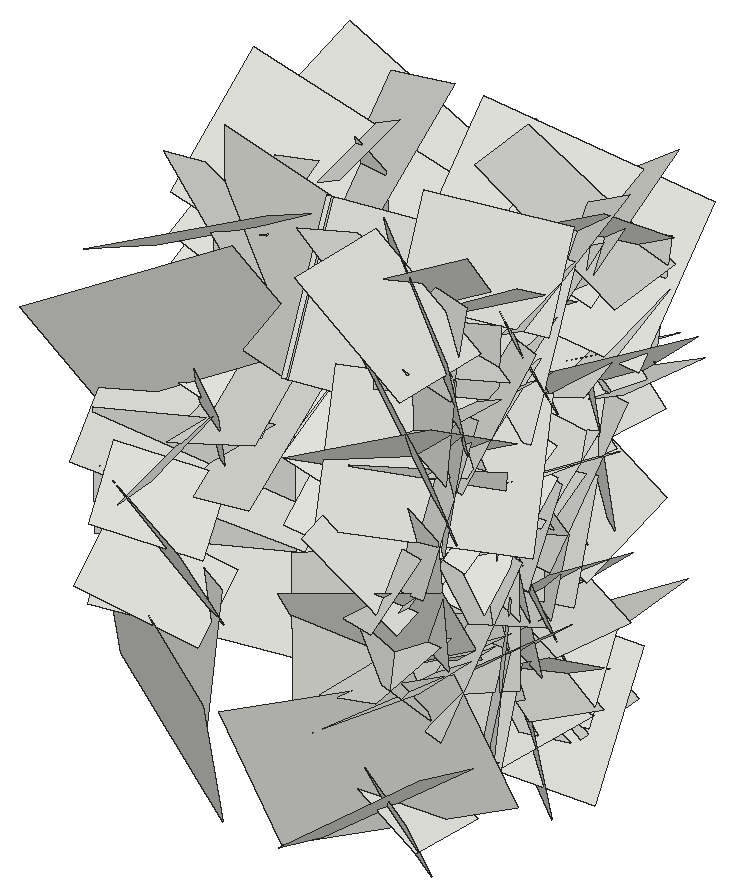
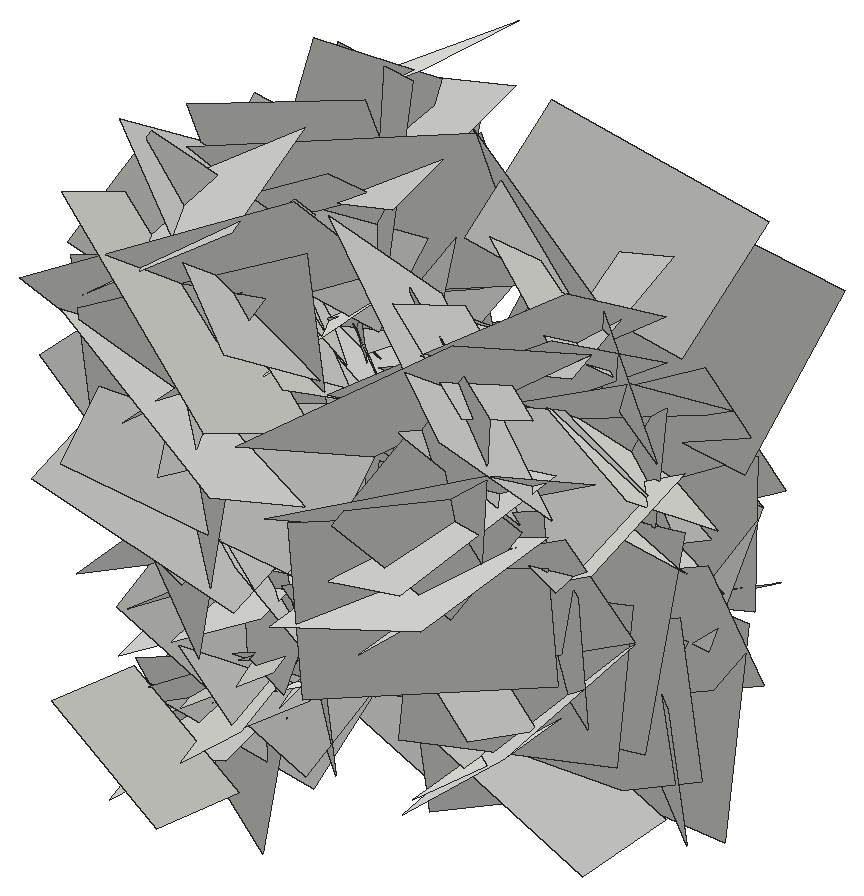
# SketchUp Ruby script. Lengths in inches.
U = 1.inch
M = Sketchup.active_model
def pt(a) = Geom::Point3d.new(a.map { |v| v * U })
def face(e, loops, mat)
  f = e.add_face(loops[0].map { |a| pt(a) })
  loops[1..].each { |l| e.add_face(l.map { |a| pt(a) }).erase! }
  f.material = f.back_material = mat if mat
  f
end
# faces: each face lists its corners as indices into pts; further lists are holes
def faces(e, pts, list, mat = nil) = list.each { |f| face(e, (f[0].is_a?(Array) ? f : [f]).map { |l| l.map { |i| pts[i] } }, mat) }
# xy, xz, yz: faces in a plane at the given z, y or x. An outline is a flat list of corners, or four numbers for a rectangle; further outlines are holes
def ring(l) = l.size == 4 ? [[l[0], l[1]], [l[2], l[1]], [l[2], l[3]], [l[0], l[3]]] : l.each_slice(2).to_a
def flat(e, list, mat, &to3) = list.each { |f| face(e, (f[0].is_a?(Array) ? f : [f]).map { |l| ring(l).map { |u, v| to3.(u, v) } }, mat) }
def xy(e, z, list, mat = nil) = flat(e, list, mat) { |x, y| [x, y, z] }
def xz(e, y, list, mat = nil) = flat(e, list, mat) { |x, z| [x, y, z] }
def yz(e, x, list, mat = nil) = flat(e, list, mat) { |y, z| [x, y, z] }
def lines(e, pts, list) = list.each { |a, b| e.add_line(pt(pts[a]), pt(pts[b])) }
# prism: a flat outline (further loops are holes) pulled along v
def prism(e, loops, v, mat = nil)
  f = face(e, loops, mat); d = Geom::Vector3d.new(v.map { |x| x * U })
  f.pushpull(f.normal.samedirection?(d) ? d.length : -d.length)
end
def box(e, o, s, mat = nil) = prism(e, [[o, [o[0] + s[0], o[1], o[2]], [o[0] + s[0], o[1] + s[1], o[2]], [o[0], o[1] + s[1], o[2]]]], [0, 0, s[2]], mat)
def at(x, y, z, deg = 0) = Geom::Transformation.translation(pt([x, y, z])) * Geom::Transformation.rotation(ORIGIN, Z_AXIS, deg.degrees)
def axes(o, x, y, z) = Geom::Transformation.new([*x, 0, *y, 0, *z, 0, *pt(o).to_a, 1])
def part(name) = M.definitions.add(name)
# library, detail: a bought-in or finely detailed component or shape, given as its bounding box
def library(name, o, s) = part(name).tap { |d| box(d.entities, o, s) }
def detail(e, o, s) = box(e.add_group.entities, o, s)
def put(e, d, t, mat = nil) = e.add_instance(d, t).tap { |i| i.material = mat if mat }
def group(e, t, mat = nil) = e.add_group.tap { |g| g.transformation = t; g.material = mat if mat }.entities
root = M.entities
c1 = part("Component\#6")
p = [[0.01,0,0],[0,3.24,4.54],[4.32,3.24,4.54],[4.33,0,0]]
faces(c1.entities,p,[[0,1,2,3]])
put(root,c1,axes([400.91,182.25,27.43],[-0.1955,0.46825,-1.21407],[0.10064,-1.21809,-0.48422],[1.37564,0.15566,-0.13711]))
put(root,c1,axes([414.68,182.25,27.43],[0.1955,0.46825,-1.21407],[-0.10064,-1.21809,-0.48422],[-1.37564,0.15566,-0.13711]))
put(root,c1,axes([414.68,183.5625,38.07],[-0.03427,-0.86867,-0.02883],[0.01016,-0.0292,0.8692],[-0.92124,0.03199,0.01066]))
put(root,c1,axes([404.88,183.51,30.36],[0.10644,-0.42009,-0.4575],[-0.01901,-0.46521,0.42323],[-0.65811,-0.0545,-0.08622]))
put(root,c1,axes([410.71,183.51,30.36],[-0.10644,-0.42009,-0.4575],[0.01901,-0.46521,0.42323],[0.65811,-0.0545,-0.08622]))
put(root,c1,axes([404.88,179.78,31.84],[0.01485,0.68647,0.23212],[0.1576,0.2245,-0.67291],[-0.75179,0.06062,-0.13648]))
put(root,c1,axes([410.71,179.78,31.84],[-0.01485,0.68647,0.23212],[-0.1576,0.2245,-0.67291],[0.75179,0.06062,-0.13648]))
put(root,c1,axes([400.91,181.64,30.57],[0.02444,0.48831,-0.77146],[0.19424,-0.75848,-0.47462],[0.9481,0.1428,0.11713]))
put(root,c1,axes([414.68,181.64,30.57],[-0.02444,0.48831,-0.77146],[-0.19424,-0.75848,-0.47462],[-0.9481,0.1428,0.11713]))
put(root,c1,axes([404.88,183.98,26.9],[0.15473,-0.64925,-0.29626],[-0.07231,-0.3137,0.65387],[-0.75301,-0.10329,-0.12366]))
put(root,c1,axes([410.71,183.98,26.9],[-0.15473,-0.64925,-0.29626],[0.07231,-0.3137,0.65387],[0.75301,-0.10329,-0.12366]))
put(root,c1,axes([410.71,181.88,29.24],[0.0732,0.47057,-0.46808],[-0.06498,-0.46407,-0.47558],[0.70054,-0.09222,0.00479]))
put(root,c1,axes([414.68,180.55,24.45],[-0.04702,0.95483,-0.28451],[0.08229,-0.28062,-0.95386],[-1.05288,-0.06457,-0.06184]))
put(root,c1,axes([410.71,182.11,23.57],[-0.01533,0.32032,-0.55846],[0.07998,-0.55391,-0.31966],[0.67773,0.07262,0.02509]))
put(root,c1,axes([400.91,182.41,31.86],[-0.21699,-0.67676,1.03332],[0.0082,1.04669,0.68705],[1.3093,-0.11872,0.16695]))
put(root,c1,axes([414.68,182.41,31.86],[0.21699,-0.67676,1.03332],[-0.0082,1.04669,0.68705],[-1.3093,-0.11872,0.16695]))
put(root,c1,axes([414.68,180.54,27.52],[-0.00647,0.86334,-0.00303],[0.00368,-0.003,-0.86336],[-0.91514,-0.00612,-0.00345]))
put(root,c1,axes([414.68,181.12,36.49],[0.0887,0.85058,-0.45713],[-0.14057,-0.44437,-0.85112],[-1.01388,0.13603,0.07801]))
put(root,c1,axes([410.71,184.65,28.76],[0.04824,-0.62434,-0.28052],[-0.09786,-0.28417,0.61748],[0.7189,0.00321,0.10288]))
put(root,c1,axes([414.68,185.4,30.76],[0.02152,-0.00963,-1.2106],[0.23963,-1.18945,0.01326],[-1.26071,-0.22625,-0.01814]))
put(root,c1,axes([410.71,181.75,22.9],[0.07496,0.59984,0.04506],[0.05269,0.03939,-0.60235],[0.63545,-0.07402,0.04463]))
put(root,c1,axes([400.91,185.55,26.35],[0.05433,-0.24183,-1.04679],[-0.06418,-1.04696,0.23891],[1.13701,-0.04754,0.0635]))
put(root,c1,axes([414.68,185.55,26.35],[-0.05433,-0.24183,-1.04679],[0.06418,-1.04696,0.23891],[-1.13701,-0.04754,0.0635]))
put(root,c1,axes([400.91,181.98,27.65],[0.03848,-0.07343,1.06513],[0.13392,1.05855,0.06867],[1.12376,-0.12364,-0.04466]))
put(root,c1,axes([414.68,181.98,27.65],[-0.03848,-0.07343,1.06513],[-0.13392,1.05855,0.06867],[-1.12376,-0.12364,-0.04466]))
put(root,c1,axes([410.71,184.92,37.05],[0.01613,-0.13323,-0.78421],[0.01491,-0.78419,0.1335],[0.84304,0.01642,0.01265]))
put(root,c1,axes([414.68,182.91,34.72],[0.14912,-0.41506,0.98502],[0.044,0.99488,0.41329],[-1.13217,-0.016,0.1458]))
put(root,c1,axes([410.71,184.84,39.1],[0.02023,-0.20369,-0.6632],[0.11732,-0.65406,0.20407],[0.72599,0.11137,-0.0145]))
put(root,c1,axes([410.71,182.78,23.92],[-0.06221,-0.24398,0.83625],[-0.07047,0.83695,0.23952],[0.92069,0.04758,0.07484]))
put(root,c1,axes([400.91,184.99,36.41],[0.13687,-0.99381,0.45239],[0.15227,0.46704,0.985],[1.14738,0.05657,-0.18469]))
put(root,c1,axes([414.68,184.99,36.41],[-0.13687,-0.99381,0.45239],[-0.15227,0.46704,0.985],[-1.14738,0.05657,-0.18469]))
put(root,c1,axes([414.68,184.8,33.37],[-0.19651,0.19461,-0.78555],[0.01158,-0.80522,-0.20206],[-0.85778,-0.05545,0.17724]))
put(root,c1,axes([414.68,187.08,35.11],[0.23629,-0.52338,-1.02054],[0.13084,-1.02265,0.55142],[-1.20867,-0.21302,-0.13982]))
put(root,c1,axes([410.71,183.74,37.84],[0.08456,-0.37494,0.46177],[-0.03825,0.46199,0.38136],[0.62935,0.07846,-0.03886]))
put(root,c1,axes([404.88,183.4375,30.23],[0.10865,-0.24445,0.66529],[-0.00738,0.67183,0.24793],[-0.75127,-0.04195,0.09378]))
put(root,c1,axes([410.71,183.4375,30.23],[-0.10865,-0.24445,0.66529],[0.00738,0.67183,0.24793],[0.75127,-0.04195,0.09378]))
put(root,c1,axes([400.91,180.73,30.67],[0.05707,0.69485,1.12415],[-0.04583,1.1254,-0.69356],[1.4001,0.00851,-0.06852]))
put(root,c1,axes([414.68,180.73,30.67],[-0.05707,0.69485,1.12415],[0.04583,1.1254,-0.69356],[-1.4001,0.00851,-0.06852]))
put(root,c1,axes([410.71,183.3,35.54],[0.06853,-0.0517,0.64839],[0.02911,0.65122,0.04919],[0.68886,-0.02238,-0.06659]))
put(root,c1,axes([410.71,186.27,36.66],[-0.23271,0.08267,-1.0169],[-0.17131,-1.02986,-0.04883],[1.06781,-0.14721,-0.22945]))
put(root,c1,axes([400.91,187.29,32.09],[-0.03087,-0.89426,-0.74249],[0.26998,-0.72958,0.86873],[1.20212,0.14089,-0.21417]))
put(root,c1,axes([414.68,187.29,32.09],[0.03087,-0.89426,-0.74249],[-0.26998,-0.72958,0.86873],[-1.20212,0.14089,-0.21417]))
put(root,c1,axes([400.91,187.26,33.24],[0.066,-0.95024,-0.64083],[0.19237,-0.6255,0.94515],[1.19957,0.15259,-0.11631]))
put(root,c1,axes([414.68,187.26,33.24],[-0.066,-0.95024,-0.64083],[-0.19237,-0.6255,0.94515],[-1.19957,0.15259,-0.11631]))
put(root,c1,axes([414.68,182.86,27.86],[-0.00866,0.87216,-0.09866],[-0.12421,-0.09886,-0.86427],[-0.92206,0.00513,0.11735]))
put(root,c1,axes([410.71,186.9,33.68],[-0.12726,-0.80704,-0.07778],[0.05104,-0.08559,0.81372],[0.85791,-0.11462,-0.05995]))
put(root,c1,axes([400.91,181.61,25.33],[-0.14764,0.72138,1.18272],[0.09804,1.19088,-0.71546],[1.46521,-0.007,0.16705]))
put(root,c1,axes([414.68,181.61,25.33],[0.14764,0.72138,1.18272],[-0.09804,1.19088,-0.71546],[-1.46521,-0.007,0.16705]))
put(root,c1,axes([414.68,186.8,27.07],[0.11611,-1.02809,0.5245],[0.14127,0.5346,1.02006],[-1.21522,-0.03608,0.16869]))
put(root,c1,axes([400.91,188.1875,39.24],[0.00053,-0.50504,-1.25708],[0.1621,-1.24903,0.50186],[1.42684,0.14209,-0.05655]))
put(root,c1,axes([414.68,188.1875,39.24],[-0.00053,-0.50504,-1.25708],[-0.1621,-1.24903,0.50186],[-1.42684,0.14209,-0.05655]))
put(root,c1,axes([400.91,182.88,33.98],[0.05541,0.90127,0.55592],[0.17138,0.54328,-0.89597],[1.1093,-0.12895,0.11065]))
put(root,c1,axes([414.68,182.88,33.98],[-0.05541,0.90127,0.55592],[-0.17138,0.54328,-0.89597],[-1.1093,-0.12895,0.11065]))
put(root,c1,axes([410.71,187.74,23.43],[-0.08523,-0.9506,0.05636],[-0.09187,0.06363,0.94959],[1.00521,-0.07479,0.09156]))
put(root,c1,axes([404.88,186.02,29.02],[0.12909,0.32312,-0.64935],[0.06195,-0.66067,-0.31779],[-0.76632,0.00102,-0.13508]))
put(root,c1,axes([410.71,186.02,29.02],[-0.12909,0.32312,-0.64935],[-0.06195,-0.66067,-0.31779],[0.76632,0.00102,-0.13508]))
put(root,c1,axes([414.68,182.62,33.52],[0.16113,0.63843,0.91206],[0.00988,0.91976,-0.64538],[-1.18006,0.09488,0.11913]))
put(root,c1,axes([410.71,187.61,26.86],[-0.07932,-0.16974,-0.83453],[-0.0041,-0.83766,0.17072],[0.9027,-0.01872,-0.07255]))
put(root,c1,axes([400.91,185.29,39.56],[0.11827,0.82487,-0.51088],[0.03346,-0.51706,-0.82795],[1.02793,-0.07808,0.08573]))
put(root,c1,axes([414.68,185.29,39.56],[-0.11827,0.82487,-0.51088],[-0.03346,-0.51706,-0.82795],[-1.02793,-0.07808,0.08573]))
put(root,c1,axes([410.71,188.3,31.13],[-0.1103,-0.11339,-0.88165],[-0.13763,-0.87621,0.12802],[0.93214,-0.14279,-0.08543]))
put(root,c1,axes([410.71,184.52,38.07],[-0.06477,0.36641,0.7198],[0.11209,0.71927,-0.35717],[0.84878,-0.06703,0.10209]))
put(root,c1,axes([414.68,184.16,23.6],[-0.00632,0.19994,1.20323],[0.15077,1.19515,-0.1979],[-1.28409,0.13934,-0.02916]))
put(root,c1,axes([400.91,184.16,23.6],[0.00632,0.19994,1.20323],[-0.15077,1.19515,-0.1979],[1.28409,0.13934,-0.02916]))
put(root,c1,axes([404.88,188.74,27.6],[0.13014,-0.45431,-0.37588],[0.00674,-0.3829,0.46487],[-0.62498,-0.09873,-0.07326]))
put(root,c1,axes([410.71,188.74,27.6],[-0.13014,-0.45431,-0.37588],[-0.00674,-0.3829,0.46487],[0.62498,-0.09873,-0.07326]))
put(root,c1,axes([410.71,188.62,32.29],[-0.0866,-0.74743,0.19758],[-0.06186,0.20408,0.74787],[0.81715,-0.06376,0.07755]))
put(root,c1,axes([404.88,185.35,37.93],[0.06077,0.5182,0.40006],[-0.00909,0.40215,-0.51968],[-0.69387,0.04012,0.04185]))
put(root,c1,axes([410.71,185.35,37.93],[-0.06077,0.5182,0.40006],[0.00909,0.40215,-0.51968],[0.69387,0.04012,0.04185]))
put(root,c1,axes([400.91,189.07,22.99],[0.09993,-0.91741,-0.05408],[0.10319,-0.04408,0.91762],[0.96866,0.09934,-0.09218]))
put(root,c1,axes([414.68,189.07,22.99],[-0.09993,-0.91741,-0.05408],[-0.10319,-0.04408,0.91762],[-0.96866,0.09934,-0.09218]))
put(root,c1,axes([400.91,186.51,25.44],[-0.00901,-0.3677,1.34811],[0.26845,1.32541,0.3631],[1.45667,-0.24653,-0.05858]))
put(root,c1,axes([414.68,186.51,25.44],[0.00901,-0.3677,1.34811],[-0.26845,1.32541,0.3631],[-1.45667,-0.24653,-0.05858]))
put(root,c1,axes([400.91,184.85,32.98],[-0.15473,1.07562,-0.16592],[0.16403,-0.14519,-1.07739],[1.14193,0.1666,0.13228]))
put(root,c1,axes([414.68,184.85,32.98],[0.15473,1.07562,-0.16592],[-0.16403,-0.14519,-1.07739],[-1.14193,0.1666,0.13228]))
put(root,c1,axes([400.91,189.26,31.29],[0.07003,-0.18149,-1.00879],[0.05402,-1.00905,0.18487],[1.08514,0.06195,0.0559]))
put(root,c1,axes([414.68,189.26,31.29],[-0.07003,-0.18149,-1.00879],[-0.05402,-1.00905,0.18487],[-1.08514,0.06195,0.0559]))
put(root,c1,axes([414.68,185.86,28.71],[0.06844,0.29244,0.76285],[-0.17475,0.75415,-0.27515],[-0.84819,-0.13178,0.11824]))
put(root,c1,axes([414.68,187.32,34.27],[-0.05201,-0.4187,0.7383],[0.02779,0.73844,0.42051],[-0.89926,0.04704,-0.0297]))
put(root,c1,axes([414.68,191.48,24.4],[0.24044,-0.84726,-0.84182],[0.11443,-0.83882,0.87332],[-1.26085,-0.2377,-0.08127]))
put(root,c1,axes([414.68,186.85,26],[-0.04759,0.74401,-0.43208],[-0.09551,-0.43435,-0.73856],[-0.90698,0.0067,0.10045]))
put(root,c1,axes([414.68,189.58,22.99],[0.08755,-0.94666,0.34405],[0.04779,0.34833,0.94763],[-1.06661,-0.0621,0.0707]))
put(root,c1,axes([414.68,186.99,20.26],[-0.04681,-0.17583,0.86867],[0.05724,0.86759,0.17835],[-0.93771,0.06173,-0.03248]))
put(root,c1,axes([400.91,190.19,31.82],[0.07854,-1.04848,0.11995],[-0.05802,0.11627,1.05008],[1.11713,0.07975,0.0461]))
put(root,c1,axes([414.68,190.19,31.82],[-0.07854,-1.04848,0.11995],[0.05802,0.11627,1.05008],[-1.11713,0.07975,0.0461]))
put(root,c1,axes([400.91,187.65,25.55],[0.14301,-0.32766,0.90945],[0.11586,0.91755,0.31436],[1.01811,-0.05839,-0.16352]))
put(root,c1,axes([414.68,187.65,25.55],[-0.14301,-0.32766,0.90945],[-0.11586,0.91755,0.31436],[-1.01811,-0.05839,-0.16352]))
put(root,c1,axes([400.91,186.92,28.87],[0.11772,1.08189,-0.3436],[-0.18933,-0.32428,-1.0788],[1.18826,-0.15885,-0.13785]))
put(root,c1,axes([414.68,186.92,28.87],[-0.11772,1.08189,-0.3436],[0.18933,-0.32428,-1.0788],[-1.18826,-0.15885,-0.13785]))
put(root,c1,axes([414.68,186.48,30.64],[-0.03295,0.70699,0.47041],[-0.18441,0.45544,-0.69599],[-0.88105,-0.12176,0.12808]))
put(root,c1,axes([400.91,185.59,36.56],[0.07365,1.00309,0.56692],[0.00038,0.56794,-1.00493],[1.22135,-0.06067,-0.03387]))
put(root,c1,axes([414.68,185.59,36.56],[-0.07365,1.00309,0.56692],[-0.00038,0.56794,-1.00493],[-1.22135,-0.06067,-0.03387]))
put(root,c1,axes([410.71,189.49,31],[-0.19159,0.03614,-0.77666],[0.1449,-0.78347,-0.06827],[0.81131,0.14846,-0.17121]))
put(root,c1,axes([414.68,189.24,21.76],[-0.15995,-0.688,0.38857],[0.02017,0.39231,0.70202],[-0.83731,0.14088,-0.05731]))
put(root,c1,axes([410.71,186.98,23.44],[-0.07046,0.41434,0.63319],[0.10971,0.63463,-0.40442],[0.79457,-0.05088,0.11199]))
put(root,c1,axes([414.68,190.89,25.45],[0.07637,-0.93381,0.1535],[-0.06656,0.14888,0.93522],[-1.00091,-0.08115,-0.05048]))
put(root,c1,axes([410.71,188.48,31.6],[0.00806,0.51701,-0.38199],[0.06142,-0.38101,-0.51453],[0.67861,0.02834,0.0511]))
put(root,c1,axes([400.91,185.63,37.94],[-0.10296,1.07287,0.66666],[-0.13207,0.65722,-1.07584],[1.33238,0.14805,-0.05512]))
put(root,c1,axes([414.68,185.63,37.94],[0.10296,1.07287,0.66666],[0.13207,0.65722,-1.07584],[-1.33238,0.14805,-0.05512]))
put(root,c1,axes([404.88,191.07,24.72],[0.08022,-0.60182,-0.03468],[0.03515,-0.03074,0.60586],[-0.63802,-0.07736,0.02902]))
put(root,c1,axes([410.71,191.07,24.72],[-0.08022,-0.60182,-0.03468],[-0.03515,-0.03074,0.60586],[0.63802,-0.07736,0.02902]))
put(root,c1,axes([414.68,187.18,35.87],[0.21905,1.32848,-0.23139],[0.18572,-0.25856,-1.32798],[-1.41727,0.17144,-0.20979]))
put(root,c1,axes([410.71,188.01,25.87],[-0.18323,0.88768,-0.1275],[-0.06793,-0.14175,-0.89995],[0.94816,0.16139,-0.08912]))
put(root,c1,axes([404.88,188.41,35.3125],[-0.03073,0.48255,0.4704],[0.10717,0.46862,-0.47449],[-0.70624,0.05011,-0.09248]))
put(root,c1,axes([410.71,188.41,35.3125],[0.03073,0.48255,0.4704],[-0.10717,0.46862,-0.47449],[0.70624,0.05011,-0.09248]))
put(root,c1,axes([400.91,186.91,28.91],[-0.08475,0.77289,1.06783],[0.0494,1.07079,-0.77154],[1.39641,0.00903,0.0921]))
put(root,c1,axes([414.68,186.91,28.91],[0.08475,0.77289,1.06783],[-0.0494,1.07079,-0.77154],[-1.39641,0.00903,0.0921]))
put(root,c1,axes([410.71,187.84,31.26],[0.01205,0.8882,0.30464],[-0.22592,0.29915,-0.86424],[0.96935,0.05868,-0.20521]))
put(root,c1,axes([404.88,188.83,29.07],[0.04972,0.59189,0.16701],[0.02122,0.16593,-0.59371],[-0.65156,0.05057,-0.00659]))
put(root,c1,axes([410.71,188.83,29.07],[-0.04972,0.59189,0.16701],[-0.02122,0.16593,-0.59371],[0.65156,0.05057,-0.00659]))
put(root,c1,axes([414.68,189.53,40.3125],[0.07096,0.70634,-0.4758],[-0.12627,-0.46481,-0.70678],[-0.89387,0.12173,0.06207]))
put(root,c1,axes([410.71,188.23,41.22],[-0.26749,1.02168,-0.17372],[0.00845,-0.17688,-1.05183],[1.0985,0.25014,-0.03421]))
put(root,c1,axes([404.88,188.93,38.32],[0.06934,0.59373,0.25],[-0.00198,0.25145,-0.59671],[-0.68287,0.05956,0.02711]))
put(root,c1,axes([410.71,188.93,38.32],[-0.06934,0.59373,0.25],[0.00198,0.25145,-0.59671],[0.68287,0.05956,0.02711]))
put(root,c1,axes([414.68,192.58,32.17],[-0.11188,-0.86522,-0.03173],[0.14554,-0.04829,0.85998],[-0.90613,0.09907,0.14204]))
put(root,c1,axes([400.91,192.86,38.11],[0.10772,-0.0541,-1.0459],[0.04447,-1.04976,0.05837],[1.10925,0.04734,0.09923]))
put(root,c1,axes([414.68,192.86,38.11],[-0.10772,-0.0541,-1.0459],[-0.04447,-1.04976,0.05837],[-1.10925,0.04734,0.09923]))
put(root,c1,axes([400.91,194.96,38.36],[-0.08597,-0.96025,-0.92678],[-0.03419,-0.92681,0.9631],[1.41421,-0.08078,-0.03305]))
put(root,c1,axes([414.68,194.96,38.36],[0.08597,-0.96025,-0.92678],[0.03419,-0.92681,0.9631],[-1.41421,-0.08078,-0.03305]))
put(root,c1,axes([400.91,190.14,35.27],[0.30668,1.10496,-0.445],[0.14325,-0.48543,-1.11748],[1.25452,-0.21469,0.23639]))
put(root,c1,axes([414.68,190.14,35.27],[-0.30668,1.10496,-0.445],[-0.14325,-0.48543,-1.11748],[-1.25452,-0.21469,0.23639]))
put(root,c1,axes([414.68,188.57,34.3],[0.02784,1.05016,0.5271],[-0.1514,0.52617,-1.0412],[-1.23628,-0.04079,0.13938]))
put(root,c1,axes([400.91,188.57,34.3],[-0.02784,1.05016,0.5271],[0.1514,0.52617,-1.0412],[1.23628,-0.04079,0.13938]))
put(root,c1,axes([414.68,190.1,29],[-0.15352,-0.05709,1.12322],[0.06907,1.13017,0.06585],[-1.19015,0.07295,-0.14107]))
put(root,c1,axes([400.91,190.1,29],[0.15352,-0.05709,1.12322],[-0.06907,1.13017,0.06585],[1.19015,0.07295,-0.14107]))
put(root,c1,axes([400.91,188.72,38.18],[0.108,1.17484,0.54266],[-0.09899,0.5496,-1.17232],[1.36819,-0.05298,-0.12766]))
put(root,c1,axes([414.68,188.72,38.18],[-0.108,1.17484,0.54266],[0.09899,0.5496,-1.17232],[-1.36819,-0.05298,-0.12766]))
put(root,c1,axes([404.88,191.45,35.51],[0.13227,0.51495,-0.41011],[0.00116,-0.41758,-0.52399],[-0.6978,0.09692,-0.07861]))
put(root,c1,axes([410.71,191.45,35.51],[-0.13227,0.51495,-0.41011],[-0.00116,-0.41758,-0.52399],[0.6978,0.09692,-0.07861]))
put(root,c1,axes([400.91,190.5,33.59],[0.11278,1.05886,-0.21225],[0.21462,-0.22906,-1.04119],[1.12442,-0.06248,0.22002]))
put(root,c1,axes([414.68,190.5,33.59],[-0.11278,1.05886,-0.21225],[-0.21462,-0.22906,-1.04119],[-1.12442,-0.06248,0.22002]))
put(root,c1,axes([404.88,193.29,29.97],[-0.02765,-0.60791,0.13872],[0.08921,0.13414,0.60366],[-0.6549,0.04394,0.07638]))
put(root,c1,axes([410.71,193.29,29.97],[0.02765,-0.60791,0.13872],[-0.08921,0.13414,0.60366],[0.6549,0.04394,0.07638]))
put(root,c1,axes([410.71,194.3125,23.26],[-0.02367,-0.75059,-0.08188],[0.02978,-0.08269,0.75031],[0.79979,-0.01914,-0.03036]))
